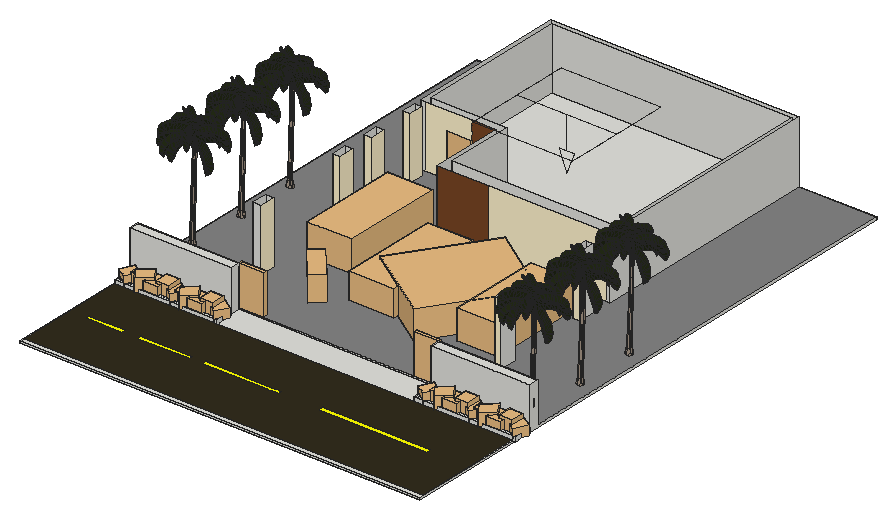
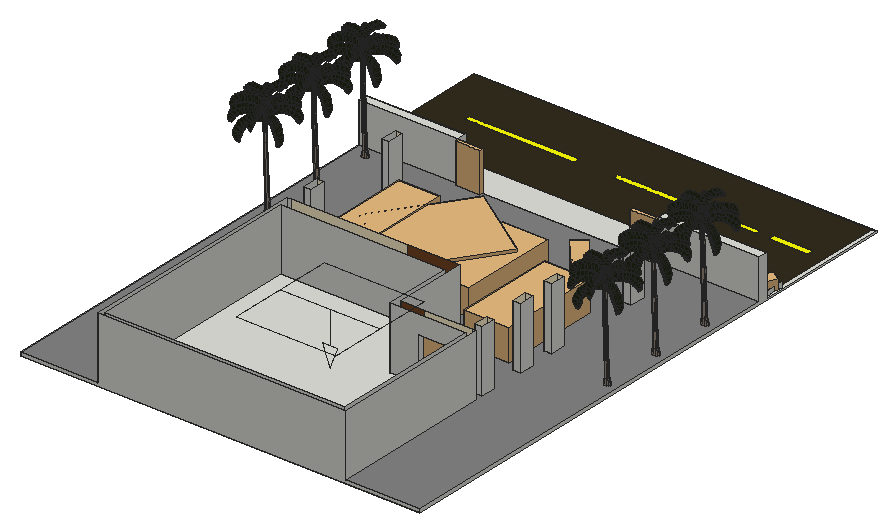
# SketchUp Ruby script. Lengths in inches.
U = 1.inch
M = Sketchup.active_model
def pt(a) = Geom::Point3d.new(a.map { |v| v * U })
def face(e, loops, mat)
  f = e.add_face(loops[0].map { |a| pt(a) })
  loops[1..].each { |l| e.add_face(l.map { |a| pt(a) }).erase! }
  f.material = f.back_material = mat if mat
  f
end
# faces: each face lists its corners as indices into pts; further lists are holes
def faces(e, pts, list, mat = nil) = list.each { |f| face(e, (f[0].is_a?(Array) ? f : [f]).map { |l| l.map { |i| pts[i] } }, mat) }
# xy, xz, yz: faces in a plane at the given z, y or x. An outline is a flat list of corners, or four numbers for a rectangle; further outlines are holes
def ring(l) = l.size == 4 ? [[l[0], l[1]], [l[2], l[1]], [l[2], l[3]], [l[0], l[3]]] : l.each_slice(2).to_a
def flat(e, list, mat, &to3) = list.each { |f| face(e, (f[0].is_a?(Array) ? f : [f]).map { |l| ring(l).map { |u, v| to3.(u, v) } }, mat) }
def xy(e, z, list, mat = nil) = flat(e, list, mat) { |x, y| [x, y, z] }
def xz(e, y, list, mat = nil) = flat(e, list, mat) { |x, z| [x, y, z] }
def yz(e, x, list, mat = nil) = flat(e, list, mat) { |y, z| [x, y, z] }
def lines(e, pts, list) = list.each { |a, b| e.add_line(pt(pts[a]), pt(pts[b])) }
# prism: a flat outline (further loops are holes) pulled along v
def prism(e, loops, v, mat = nil)
  f = face(e, loops, mat); d = Geom::Vector3d.new(v.map { |x| x * U })
  f.pushpull(f.normal.samedirection?(d) ? d.length : -d.length)
end
def box(e, o, s, mat = nil) = prism(e, [[o, [o[0] + s[0], o[1], o[2]], [o[0] + s[0], o[1] + s[1], o[2]], [o[0], o[1] + s[1], o[2]]]], [0, 0, s[2]], mat)
def at(x, y, z, deg = 0) = Geom::Transformation.translation(pt([x, y, z])) * Geom::Transformation.rotation(ORIGIN, Z_AXIS, deg.degrees)
def axes(o, x, y, z) = Geom::Transformation.new([*x, 0, *y, 0, *z, 0, *pt(o).to_a, 1])
def part(name) = M.definitions.add(name)
# library, detail: a bought-in or finely detailed component or shape, given as its bounding box
def library(name, o, s) = part(name).tap { |d| box(d.entities, o, s) }
def detail(e, o, s) = box(e.add_group.entities, o, s)
def put(e, d, t, mat = nil) = e.add_instance(d, t).tap { |i| i.material = mat if mat }
def group(e, t, mat = nil) = e.add_group.tap { |g| g.transformation = t; g.material = mat if mat }.entities
root = M.entities
M.materials.add("Manila2").color = [36, 43, 22]
M.materials.add("ManilaTruck").color = [158, 143, 128]
M.materials.add("Material__1").color = [95, 70, 46]
M.materials.add("[Color D01]").color = [255, 242, 204]
M.materials.add("[Color_D24]").color = [51, 45, 30]
M.materials.add("[Color_E01]").color = [255, 255, 0]
M.materials.add("[Tile Grey]").color = [132, 132, 132]
M.materials.add("[Wood Veneer 01]").color = [120, 70, 37]
c1 = part("P_trunck")
xz(c1.entities,2.71,[[7.39,73.15,8.49,73.15,9.26,91.63,8.16,91.63]],"ManilaTruck")
xz(c1.entities,6.09,[[3.91,10.2,7.39,73.15,8.49,73.15,5.33,10.2],[7.39,73.15,8.16,91.63,9.26,91.63,8.49,73.15]],"ManilaTruck")
p = [[3.19,0,0],[3.91,1.7,10.2],[2.75,2.54,10.2],[0.88,1.68,0],[6.05,0,0],[5.33,1.7,10.2],
  [8.36,1.68,0],[6.49,2.54,10.2],[2.31,3.9,10.2],[0,4.39,0],[9.24,4.39,0],[6.93,3.9,10.2],
  [2.75,5.25,10.2],[0.88,7.11,0],[8.36,7.11,0],[6.49,5.25,10.2],[3.91,6.09,10.2],[3.19,8.79,0],
  [6.05,8.79,0],[5.33,6.09,10.2],[7.39,2.71,73.15],[6.5,3.36,73.15],[8.49,2.71,73.15],[9.38,3.36,73.15],
  [6.16,4.4,73.15],[9.72,4.4,73.15],[6.5,5.45,73.15],[9.38,5.45,73.15],[7.39,6.09,73.15],[8.49,6.09,73.15],
  [8.16,2.71,91.63],[7.27,3.36,91.63],[10.15,3.36,91.63],[9.26,2.71,91.63],[6.93,4.4,91.63],[10.49,4.4,91.63],
  [7.27,5.45,91.63],[10.15,5.45,91.63],[8.16,6.09,91.63],[9.26,6.09,91.63]]
faces(c1.entities,p,[[0,1,2,3],[4,5,1,0],[6,7,5,4],[3,2,8,9],[6,10,11,7],[8,12,13,9],[11,10,14,15],[13,12,16,17],
  [18,19,15,14],[17,16,19,18],[1,20,21,2],[5,22,20,1],[7,23,22,5],[2,21,24,8],[7,11,25,23],[8,24,26,12],
  [11,15,27,25],[12,26,28,16],[19,29,27,15],[20,30,31,21],[23,32,33,22],[31,34,24,21],[23,25,35,32],[34,36,26,24],
  [25,27,37,35],[26,36,38,28],[29,39,37,27]],"ManilaTruck")
c2 = part("halfleave")
p = [[3.15,0,0],[0.57,2.5,1.86],[4.875,1.71,0],[46.16,1.62,0],[42.0625,6.98,0],[45.79,16.25,3.85],
  [48.16,12.12,1.98],[48.16,1.62,0],[6.6,3.42,0],[-0.25,5.68,3.48],[9.02,6.6,0],[-0.31,11.68,4.96],
  [2.05,16.625,5.9],[10.99,8.52,0],[36.71,10.67,0],[41.5,21.18,5.01],[8.2,21.17,6.52],[12.96,10.44,0],
  [15.16,24.88,6.8125],[17.61,12.89,0],[31.19,13.02,0],[36.16,23.66,5.26],[19.91,24.88,6.5625],[20.53,13.55,0],
  [25.77,13.9375,0],[30.57,24.88,6.0625],[25.21,24.88,6.26]]
faces(c2.entities,p,[[0,1,2],[3,4,5],[5,6,3],[7,3,6],[2,1,8],[9,8,1],[8,9,10],[11,10,9],
  [11,12,10],[13,10,12],[4,14,15],[15,5,4],[12,16,13],[17,13,16],[16,18,17],[19,17,18],
  [14,20,21],[21,15,14],[18,22,19],[23,19,22],[20,24,25],[25,21,20],[22,26,23],[24,23,26],
  [26,25,24]],"Manila2")
c3 = part("palmfronmanila")
put(c3.entities,c2,axes([0,0,4.06],[1,0,0],[0,1,0],[0,0,-1]))
put(c3.entities,c2,at(0,0,4.06))
c4 = part("manilafronnew")
put(c4.entities,c3,axes([0,16.76,11.56],[1,0,0],[0,0,1],[0,-1,0]))
c5 = part("Palm tree")
put(c5.entities,c1,axes([-10.55,-3.84,0],[1.24992,0,0],[0,1.28016,0],[0,0,1.424]))
g1 = group(c5.entities,at(-43.54,-39.32,114.59))
put(g1,c4,axes([4.6,65.71,26.23],[0.53953,-0.65683,-0.22776],[0.61942,0.58508,-0.22],[0.31564,-0.02543,0.82105]))
put(g1,c4,axes([82.14,44.18,-7.44],[-0.84198,0.16366,0.22983],[-0.16944,-0.87168,0],[0.22561,-0.04385,0.85774]))
put(g1,c4,axes([74.79,11.41,2.76],[-0.448,0.77596,0],[-0.77596,-0.448,0],[0,0,0.896]))
put(g1,c4,axes([70.64,6.04,20.22],[-0.30809,0.82895,-0.08038],[-0.79676,-0.31832,-0.22889],[-0.24248,-0.00729,0.85422]))
put(g1,c4,axes([56.04,79.09,38.5],[-0.31814,-0.55104,-0.36736],[0.63629,-0.36736,0],[-0.18368,-0.31814,0.63629]))
put(g1,c4,axes([8.39,50.1,50.01],[0.44591,-0.25744,-0.51489],[0.36408,0.63061,0],[0.44591,-0.25744,0.51489]))
put(g1,c4,axes([8.53,12.03,22.52],[0.79394,0.3635,-0.23397],[-0.37632,0.82195,0],[0.21274,0.0974,0.8732]))
put(g1,c4,axes([54.07,81.55,-7.16],[-0.44094,-0.76373,0.19874],[0.78289,-0.452,0],[0.09937,0.17211,0.88188]))
put(g1,c4,axes([11.98,71.79,5.35],[0.444,-0.76903,0],[0.76903,0.444,0],[0,0,0.888]))
put(g1,c4,axes([-0.47,46.08,5.17],[0.83758,-0.34011,0],[0.34011,0.83758,0],[0,0,0.904]))
put(g1,c4,axes([35.85,3.71,-10.8],[0.42686,0.73934,0.2973],[-0.78289,0.452,0],[-0.14865,-0.25747,0.85372]))
put(g1,c4,axes([0.28,29.91,5.17],[0.904,0,0],[0,0.904,0],[0,0,0.904]))
put(g1,c4,axes([82.45,61.59,11.57],[-0.88287,-0.17622,-0.08182],[0.17259,-0.88617,0.04625],[-0.08923,0.02954,0.8991]))
put(g1,c4,axes([59.47,9.58,46.3125],[-0.10851,0.51281,-0.52416],[-0.72522,-0.15346,0],[-0.10851,0.51281,0.52416]))
c6 = part("עצי+דקל")
put(c6.entities,c5,axes([111.95,22.91,0],[1.33,0,0],[0,1.33,0],[0,0,1.33]))
put(c6.entities,c5,axes([230.0625,22.91,0],[1.33,0,0],[0,1.33,0],[0,0,1.33]))
put(c6.entities,c5,axes([348.17,22.91,0],[1.33,0,0],[0,1.33,0],[0,0,1.33]))
c7 = library("Areca palm plant",[0,0,0],[49.1,36.6,54.46])
c8 = library("Group38\#2",[14.01,28.44,-23.43],[18.58,18.32,38.89])
c9 = library("Group\#32",[-84.69,-90.07,-0.36],[176.51,175.13,171.4])
c10 = library("Group20\#1",[-20.81,-17.08,3.79],[39.86,39.43,37.51])
c11 = library("Group\#130",[-7.34,-1.2,0],[38.67,35.81,49.04])
c12 = part("Group\#35")
put(c12.entities,c7,axes([-6.2,158.41,6.08],[0.45017,-0.56191,0],[0.66137,0.52986,0],[0,0,0.72]))
put(c12.entities,c7,axes([-6.2,56.6,6.08],[0.45017,-0.56191,0],[0.66137,0.52986,0],[0,0,0.72]))
put(c12.entities,c8,axes([-4.1,-1.15,28.17],[0.8848,0,0],[0,0.94674,0],[0,0,0.85826]))
put(c12.entities,c8,axes([-4.1,100.66,28.17],[0.8848,0,0],[0,0.94674,0],[0,0,0.85826]))
g2 = group(c12.entities,at(0,0,0))
xy(g2,0,[[0,0,6,234.8],[30,0,36,234.8]])
xy(g2,3,[[6,0,30,234.8]])
xy(g2,7,[[6,5,30,229.8]],"Material__1")
xy(g2,15,[[[0,0,36,234.8],[6,5,30,229.8]]])
xz(g2,0,[[0,0,6,0,6,3,30,3,30,0,36,0,36,15,0,15]])
xz(g2,5,[[6,7,30,15]])
xz(g2,229.8,[[6,7,30,15]])
xz(g2,234.8,[[0,0,0,15,36,15,36,0,30,0,30,3,6,3,6,0]])
yz(g2,0,[[0,0,234.8,15]])
yz(g2,6,[[0,0,234.8,3],[5,7,229.8,15]])
yz(g2,30,[[0,0,234.8,3],[5,7,229.8,15]])
yz(g2,36,[[0,0,234.8,15]])
put(c12.entities,c9,axes([17.19,121.23,6.07],[-0.08133,-0.14087,0],[0.14087,-0.08133,0],[0,0,0.1725]))
put(c12.entities,c9,axes([14.93,173.12,6.05],[-0.04961,-0.08593,0],[0.08593,-0.04961,0],[0,0,0.10522]))
put(c12.entities,c10,axes([18.97,79.98,4.77],[0,0.85,0],[-0.85,0,0],[0,0,0.85]))
put(c12.entities,c9,axes([17.19,223.04,6.07],[-0.08133,-0.14087,0],[0.14087,-0.08133,0],[0,0,0.1725]))
put(c12.entities,c9,axes([14.93,71.3,6.05],[-0.04961,-0.08593,0],[0.08593,-0.04961,0],[0,0,0.10522]))
put(c12.entities,c11,axes([24.9375,191.72,8],[0,0.79,0],[-0.79,0,0],[0,0,0.79]))
put(c12.entities,c10,axes([18.97,181.79,4.77],[0,0.85,0],[-0.85,0,0],[0,0,0.85]))
put(c12.entities,c11,axes([24.9375,89.91,8],[0,0.79,0],[-0.79,0,0],[0,0,0.79]))
put(c12.entities,c9,axes([14.93,91.37,6.05],[-0.04961,-0.08593,0],[0.08593,-0.04961,0],[0,0,0.10522]))
put(c12.entities,c9,axes([14.93,145.87,6.05],[-0.04961,-0.08593,0],[0.08593,-0.04961,0],[0,0,0.10522]))
put(c12.entities,c9,axes([17.19,15.79,6.07],[-0.08133,-0.14087,0],[0.14087,-0.08133,0],[0,0,0.1725]))
put(c12.entities,c9,axes([14.93,193.18,6.05],[-0.04961,-0.08593,0],[0.08593,-0.04961,0],[0,0,0.10522]))
put(c12.entities,c9,axes([14.93,44.05,6.05],[-0.04961,-0.08593,0],[0.08593,-0.04961,0],[0,0,0.10522]))
c13 = library("Group\#36",[0,0,0],[85.51,189.4,58.01])
c14 = part("2022 BMW i4")
put(c14.entities,c13,axes([0,0,0],[5,0,0],[0,5,0],[0,0,5]))
c15 = library("SLIDING GATE",[0,0,0],[90.55,6.89,64.23])
c16 = library("BMW 8 Series M850i 2019",[-14.25,0.77,-0.16],[87.38,190.63,50.87])
c17 = library("2008 BMW M3 e90",[0,0,0],[79.3,179.66,56.06])
c18 = library("BMW+S1000R",[-41.95,-39.66,31.8],[27.64,81.64,47.06])
c19 = library("元件\#5",[-4.39,0,0],[5.37,35.83,90.55])
c20 = part("Untitled (4)")
xy(c20.entities,0,[[[0,0,732.28,1478.74],[337.5,926.31,374.12,1332.21],[336.78,491.28,371.03,780.65],[337.46,251.99,371.32,448.45],[335.4,57.93,372.8,197.6875]]],"[Color_D24]")
xy(c20.entities,0,[[335.4,57.93,372.8,197.6875],[337.46,251.99,371.32,448.45],[336.78,491.28,371.03,780.65],[337.5,926.31,374.12,1332.21]],"[Color_E01]")
c21 = library("002+Bmw+M4+++mat3.4+2017",[-252.8,19.48,9.01],[196.94,171.32,55.15])
c22 = part("Group74\#1")
p = [[0,0,0],[0,0,-62.84],[-14.84,0,-62.84],[96.59,-106.85,0],[-96.59,-106.85,0],[96.59,106.85,0],
  [96.59,0,0],[-96.59,106.85,0],[14.84,0,-62.84],[-96.59,0,0],[0,0,-101.72]]
lines(c22.entities,p,[[0,1],[1,2],[3,4],[5,6],[7,5],[1,8],[9,0],[0,6],[8,10],[4,9],[6,3],[2,10],
  [9,7]])
c23 = part("Rectangle Light\#1")
put(c23.entities,c22,at(0,0,0))
xy(root,0,[[33.625,0,807.5,1103.3125]])
xy(root,3,[[33.625,0,807.5,0,807.5,265.25,616.39,265.25,616.39,283.67,230.35,283.67,230.35,265.25,33.625,265.25]])
xy(root,6,[[177.75,383.3125,193.125,412.64],[644.75,383.3125,657.75,415.125],[644.75,572.73,657.75,604.54],[177.75,575.25,192.5,604.58],[177.75,651.6,192.5,680.93],
  [332.57,669.6875,650.24,669.6875,650.24,1095.81,185.26,1095.81,185.26,802.9375,332.57,802.9375],[177.75,744.25,192.5,773.58]])
xy(root,6,[[[33.625,283.67,807.5,283.67,807.5,1103.3125,657.75,1103.3125,657.75,645.5,324.13,645.5,324.13,788.13,276.23,788.13,276.23,802.9375,228.23,802.9375,228.23,788.13,177.75,788.13,177.75,1103.3125,33.625,1103.3125],[177.75,383.3125,193.125,412.64],[177.75,575.25,192.5,604.58],[177.75,651.6,192.5,680.93],[177.75,744.25,192.5,773.58],[644.75,572.73,657.75,604.54],[644.75,383.3125,657.75,415.125]]],"[Tile Grey]")
xy(root,82.9375,[[33.625,265.25,230.35,283.67],[616.39,265.25,807.5,283.67]])
xy(root,90,[[228.23,788.13,276.23,802.9375]])
xz(root,0,[[33.625,0,807.5,3]])
xz(root,265.25,[[33.625,3,230.35,82.9375],[616.39,3,807.5,82.9375]])
xz(root,283.67,[[230.35,3,616.39,6],[33.625,6,230.35,82.9375],[616.39,6,807.5,82.9375]])
xz(root,383.3125,[[177.75,6,193.125,126]])
xz(root,383.3125,[[644.75,6,657.75,126]],"[Color D01]")
xz(root,412.64,[[177.75,6,193.125,126]])
xz(root,415.125,[[644.75,6,657.75,126]])
xz(root,572.73,[[644.75,6,657.75,126]],"[Color D01]")
xz(root,575.25,[[177.75,6,192.5,126]],"[Color D01]")
xz(root,604.54,[[644.75,6,657.75,126]])
xz(root,604.58,[[177.75,6,192.5,126]])
xz(root,645.5,[[650.24,6,657.75,126]])
xz(root,645.5,[[424.17,6,650.24,126]],"[Color D01]")
xz(root,645.5,[[324.13,6,424.17,126]],"[Wood Veneer 01]")
xz(root,651.6,[[177.75,6,192.5,126]],"[Color D01]")
xz(root,669.6875,[[332.57,6,650.24,126]])
xz(root,680.93,[[177.75,6,192.5,126]])
xz(root,744.25,[[177.75,6,192.5,126]],"[Color D01]")
xz(root,773.58,[[177.75,6,192.5,126]])
xz(root,788.13,[[177.75,6,185.26,126]])
xz(root,788.13,[[185.26,6,228.23,6,228.23,90,276.23,90,276.23,126,185.26,126]],"[Color D01]")
xz(root,788.13,[[276.23,6,324.13,126]],"[Wood Veneer 01]")
xz(root,802.9375,[[185.26,6,185.26,126,332.57,126,332.57,6,276.23,6,276.23,90,228.23,90,228.23,6]])
xz(root,1095.81,[[185.26,6,650.24,126]])
xz(root,1103.3125,[[33.625,0,33.625,6,177.75,6,177.75,126,657.75,126,657.75,6,807.5,6,807.5,0]])
yz(root,33.625,[[0,0,0,3,265.25,3,265.25,82.9375,283.67,82.9375,283.67,6,1103.3125,6,1103.3125,0]])
yz(root,177.75,[[383.3125,6,412.64,126],[575.25,6,604.58,126],[651.6,6,680.93,126],[744.25,6,773.58,126],[788.13,6,1103.3125,126]])
yz(root,185.26,[[802.9375,6,1095.81,126]])
yz(root,192.5,[[575.25,6,604.58,126],[651.6,6,680.93,126],[744.25,6,773.58,126]],"[Color D01]")
yz(root,193.125,[[383.3125,6,412.64,126]],"[Color D01]")
yz(root,228.23,[[788.13,6,802.9375,90]])
yz(root,230.35,[[265.25,3,283.67,82.9375]])
yz(root,276.23,[[788.13,6,802.9375,90]])
yz(root,324.13,[[645.5,6,788.13,126]])
yz(root,332.57,[[669.6875,6,802.9375,126]])
yz(root,616.39,[[265.25,3,283.67,82.9375]])
yz(root,644.75,[[383.3125,6,415.125,126],[572.73,6,604.54,126]])
yz(root,650.24,[[669.6875,6,1095.81,126]])
yz(root,657.75,[[383.3125,6,415.125,126],[572.73,6,604.54,126],[645.5,6,1103.3125,126]])
yz(root,807.5,[[0,0,1103.3125,0,1103.3125,6,283.67,6,283.67,82.9375,265.25,82.9375,265.25,3,0,3]])
put(root,c6,at(804.02,199.25,-1.6,90))
put(root,c6,at(80.06,282.62,-1.6,90))
put(root,c12,axes([37.03,258.7,3],[0,-0.952,0],[0.84,0,0],[0,0,0.61]))
put(root,c12,axes([615.85,258.7,3],[0,-0.952,0],[0.84,0,0],[0,0,0.61]))
put(root,c14,axes([210.6,471.86,6],[0.20577,0,0],[0,0.20577,0],[0,0,0.20577]))
put(root,c15,axes([230.35,283.67,6],[0.52,0,0],[0,1,0],[0,0,1.19782]))
put(root,c16,at(418.74,595.98,6.16,180))
put(root,c17,at(550.61,409.91,6))
put(root,c18,at(308.56,418.08,-25.8,40.1))
put(root,c15,axes([568.66,283.67,6],[0.52,0,0],[0,1,0],[0,0,1.19782]))
put(root,c19,axes([228.23,788.5,6],[0,-1,0],[1.33978,0,0],[0,0,0.92765]))
put(root,c20,axes([38.56,222.3125,6],[0,-0.2964,0],[0.52,0,0],[0,0,0.52]))
put(root,c21,at(658.97,565.32,-2.8125,55.8))
put(root,c23,axes([384.93,882.59,131.99],[-1,0,0],[0,1,0],[0,0,1]))
